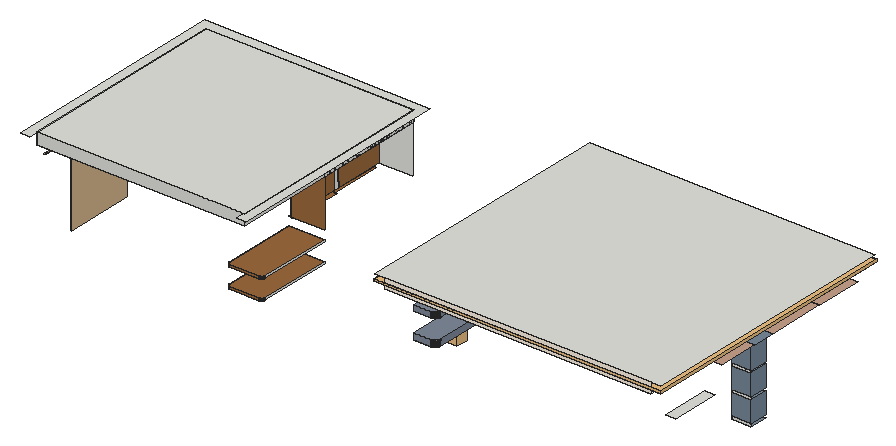
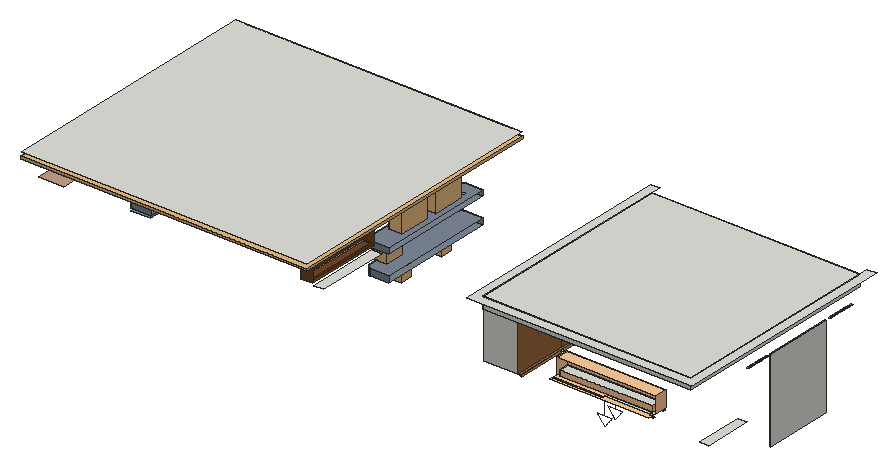
# SketchUp Ruby script. Lengths in inches.
U = 1.inch
M = Sketchup.active_model
def pt(a) = Geom::Point3d.new(a.map { |v| v * U })
def face(e, loops, mat)
  f = e.add_face(loops[0].map { |a| pt(a) })
  loops[1..].each { |l| e.add_face(l.map { |a| pt(a) }).erase! }
  f.material = f.back_material = mat if mat
  f
end
# faces: each face lists its corners as indices into pts; further lists are holes
def faces(e, pts, list, mat = nil) = list.each { |f| face(e, (f[0].is_a?(Array) ? f : [f]).map { |l| l.map { |i| pts[i] } }, mat) }
# xy, xz, yz: faces in a plane at the given z, y or x. An outline is a flat list of corners, or four numbers for a rectangle; further outlines are holes
def ring(l) = l.size == 4 ? [[l[0], l[1]], [l[2], l[1]], [l[2], l[3]], [l[0], l[3]]] : l.each_slice(2).to_a
def flat(e, list, mat, &to3) = list.each { |f| face(e, (f[0].is_a?(Array) ? f : [f]).map { |l| ring(l).map { |u, v| to3.(u, v) } }, mat) }
def xy(e, z, list, mat = nil) = flat(e, list, mat) { |x, y| [x, y, z] }
def xz(e, y, list, mat = nil) = flat(e, list, mat) { |x, z| [x, y, z] }
def yz(e, x, list, mat = nil) = flat(e, list, mat) { |y, z| [x, y, z] }
def lines(e, pts, list) = list.each { |a, b| e.add_line(pt(pts[a]), pt(pts[b])) }
# prism: a flat outline (further loops are holes) pulled along v
def prism(e, loops, v, mat = nil)
  f = face(e, loops, mat); d = Geom::Vector3d.new(v.map { |x| x * U })
  f.pushpull(f.normal.samedirection?(d) ? d.length : -d.length)
end
def box(e, o, s, mat = nil) = prism(e, [[o, [o[0] + s[0], o[1], o[2]], [o[0] + s[0], o[1] + s[1], o[2]], [o[0], o[1] + s[1], o[2]]]], [0, 0, s[2]], mat)
def at(x, y, z, deg = 0) = Geom::Transformation.translation(pt([x, y, z])) * Geom::Transformation.rotation(ORIGIN, Z_AXIS, deg.degrees)
def axes(o, x, y, z) = Geom::Transformation.new([*x, 0, *y, 0, *z, 0, *pt(o).to_a, 1])
def part(name) = M.definitions.add(name)
# library, detail: a bought-in or finely detailed component or shape, given as its bounding box
def library(name, o, s) = part(name).tap { |d| box(d.entities, o, s) }
def detail(e, o, s) = box(e.add_group.entities, o, s)
def put(e, d, t, mat = nil) = e.add_instance(d, t).tap { |i| i.material = mat if mat }
def group(e, t, mat = nil) = e.add_group.tap { |g| g.transformation = t; g.material = mat if mat }.entities
root = M.entities
M.materials.add("Plywood B 50cm").color = [193, 159, 125]
M.materials.add("[0009_Linen]").color = [197, 160, 138]
M.materials.add("[0035_Tan]").color = [210, 180, 140]
M.materials.add("[0110_LightSlateGray]").color = [127, 136, 153]
M.materials.add("[0110_LightSlateGray]1").color = [119, 136, 153]
M.materials.add("[Color C02]").color = [255, 204, 153]
M.materials.add("[Color D01]").color = [255, 242, 228]
M.materials.add("[Fencing Lattice Natural]").color = [179, 148, 127]
M.materials.add("[Wood Floor]").color = [155, 105, 61]
M.materials.add("[Wood Veneer 01]").color = [120, 70, 37]
c1 = library("Spot Light\#1",[-5.1,-5.1,-11.05],[10.2,10.2,11.05])
c2 = library("Spot Light\#3",[-5.1,-5.1,-11.05],[10.2,10.2,11.05])
c3 = library("Spot Light\#2",[-5.1,-5.1,-11.05],[10.2,10.2,11.05])
c4 = part("Group30\#1")
p = [[0,0,0],[0,0,-13.91],[-6.7,0,-13.91],[43.59,-1.45,0],[-43.59,-1.45,0],[43.59,1.45,0],
  [43.59,0,0],[-43.59,1.45,0],[6.7,0,-13.91],[-43.59,0,0],[0,0,-22.52]]
lines(c4.entities,p,[[0,1],[1,2],[3,4],[5,6],[7,5],[1,8],[9,0],[0,6],[8,10],[4,9],[6,3],[2,10],
  [9,7]])
c5 = part("Rectangle Light\#1")
put(c5.entities,c4,at(0,0,0))
c6 = part("Group7\#1")
p = [[0,0,0],[0,0,-13.88],[-6.7,0,-13.88],[43.59,-1.36,0],[-43.59,-1.36,0],[43.59,1.36,0],
  [43.59,0,0],[-43.59,1.36,0],[6.7,0,-13.88],[-43.59,0,0],[0,0,-22.48]]
lines(c6.entities,p,[[0,1],[1,2],[3,4],[5,6],[7,5],[1,8],[9,0],[0,6],[8,10],[4,9],[6,3],[2,10],
  [9,7]])
c7 = part("Rectangle Light")
put(c7.entities,c6,at(0,0,0))
c8 = library("Decorative Puppy 209 004",[-5.43,-3.24,0],[10.86,6.48,10.94])
c9 = library("Books 120 040",[-9.2,-4.08,-0.03],[18.37,8.13,11.52])
c10 = library("Dome Light",[-12,-12,0],[24,24,12])
c11 = library("Mesh Light\#4",[-0.5,-0.5,-0.1],[1,1,0.2])
c12 = library("Group\#10",[-0.5,-0.5,2.25],[131.75,125.15,1.375])
box(root,[8.12,10.37,154.875],[183.2,186.7,9.875])
xy(root,71.0625,[[8.12,47.65,9.43,108.01]])
xy(root,76.9375,[[536.14,116.57,553.2,132.48]],"[0110_LightSlateGray]1")
xy(root,78.9375,[[536.14,116.57,553.2,132.48]],"[0110_LightSlateGray]1")
xy(root,86.125,[[162.88,30.24,162.49,30.26,162.11,30.34,161.73,30.46,161.38,30.64,161.06,30.86,160.76,31.11,160.5,31.41,160.28,31.74,160.11,32.09,159.98,32.46,159.91,32.84,159.88,33.24,159.88,98.61,191.32,98.61,191.32,33.18,191.29,32.79,191.22,32.42,191.1,32.05,190.93,31.71,190.71,31.39,190.46,31.1,190.17,30.84,189.85,30.63,189.5,30.46,189.14,30.34,188.76,30.26,188.38,30.24]],"[Wood Floor]")
xy(root,88.125,[[162.88,30.24,188.38,30.24,188.76,30.26,189.14,30.34,189.5,30.46,189.85,30.63,190.17,30.84,190.46,31.1,190.71,31.39,190.93,31.71,191.1,32.05,191.22,32.42,191.29,32.79,191.32,33.18,191.32,98.61,159.88,98.61,159.88,33.24,159.91,32.84,159.98,32.46,160.11,32.09,160.28,31.74,160.5,31.41,160.76,31.11,161.06,30.86,161.38,30.64,161.73,30.46,162.11,30.34,162.49,30.26]],"[Wood Floor]")
xy(root,98.06,[[536.14,116.57,553.2,132.48]],"[0110_LightSlateGray]1")
xy(root,100.06,[[536.14,116.57,553.2,132.48]],"[0110_LightSlateGray]1")
xy(root,102.15,[[[323.37,31.6,323.37,136.04,338.74,136.04,339.39,136,340.03,135.87,340.65,135.66,341.24,135.37,341.78,135.01,342.28,134.58,342.71,134.09,343.07,133.54,343.36,132.95,343.57,132.34,343.7,131.69,343.74,131.04,343.74,36.6,343.7,35.95,343.57,35.31,343.36,34.69,343.07,34.1,342.71,33.56,342.28,33.07,341.78,32.64,341.24,32.27,340.65,31.98,340.03,31.77,339.39,31.65,338.74,31.6],[335.21,103.85,336.25,103.98,337.21,104.38,338.04,105.02,338.68,105.85,339.07,106.81,339.21,107.85,339.07,108.88,338.68,109.85,338.04,110.67,337.21,111.31,336.25,111.71,335.21,111.85,334.18,111.71,333.21,111.31,332.38,110.67,331.75,109.85,331.35,108.88,331.21,107.85,331.35,106.81,331.75,105.85,332.38,105.02,333.21,104.38,334.18,103.98],[335.41,60.3125,336.29,60.48,337.1,60.87,337.78,61.46,338.28,62.2,338.58,63.05,338.64,63.94,338.48,64.82,338.09,65.63,337.5,66.3125,336.76,66.82,335.91,67.11,335.02,67.18,334.13,67.01,333.33,66.62,332.65,66.03,332.14,65.29,331.85,64.44,331.78,63.55,331.95,62.67,332.34,61.86,332.92,61.18,333.66,60.68,334.51,60.38]]],"[0110_LightSlateGray]")
xy(root,103.09,[[335.21,103.85,334.18,103.98,333.21,104.38,332.38,105.02,331.75,105.85,331.35,106.81,331.21,107.85,331.35,108.88,331.75,109.85,332.38,110.67,333.21,111.31,334.18,111.71,335.21,111.85,336.25,111.71,337.21,111.31,338.04,110.67,338.68,109.85,339.07,108.88,339.21,107.85,339.07,106.81,338.68,105.85,338.04,105.02,337.21,104.38,336.25,103.98]],"[0110_LightSlateGray]")
xy(root,103.5,[[162.88,30.24,162.49,30.26,162.11,30.34,161.73,30.46,161.38,30.64,161.06,30.86,160.76,31.11,160.5,31.41,160.28,31.74,160.11,32.09,159.98,32.46,159.91,32.84,159.88,33.24,159.88,98.61,191.32,98.61,191.32,33.24,191.29,32.84,191.22,32.46,191.09,32.09,190.92,31.74,190.7,31.41,190.44,31.11,190.15,30.86,189.82,30.64,189.47,30.46,189.1,30.34,188.71,30.26,188.32,30.24]],"[Wood Floor]")
xy(root,103.53,[[335.41,60.3125,334.51,60.38,333.66,60.68,332.92,61.18,332.34,61.86,331.95,62.67,331.78,63.55,331.85,64.44,332.14,65.29,332.65,66.03,333.33,66.62,334.13,67.01,335.02,67.18,335.91,67.11,336.76,66.82,337.5,66.3125,338.09,65.63,338.48,64.82,338.64,63.94,338.58,63.05,338.28,62.2,337.78,61.46,337.1,60.87,336.29,60.48]],"[0110_LightSlateGray]")
xy(root,105.5,[[162.88,30.24,188.32,30.24,188.71,30.26,189.1,30.34,189.47,30.46,189.82,30.64,190.15,30.86,190.44,31.11,190.7,31.41,190.92,31.74,191.09,32.09,191.22,32.46,191.29,32.84,191.32,33.24,191.32,98.61,159.88,98.61,159.88,33.24,159.91,32.84,159.98,32.46,160.11,32.09,160.28,31.74,160.5,31.41,160.76,31.11,161.06,30.86,161.38,30.64,161.73,30.46,162.11,30.34,162.49,30.26]],"[Wood Floor]")
xy(root,107.71,[[323.37,31.6,338.74,31.6,339.39,31.65,340.03,31.77,340.65,31.98,341.24,32.27,341.78,32.64,342.28,33.07,342.71,33.56,343.07,34.1,343.36,34.69,343.57,35.31,343.7,35.95,343.74,36.6,343.74,131.04,343.7,131.69,343.57,132.34,343.36,132.95,343.07,133.54,342.71,134.09,342.28,134.58,341.78,135.01,341.24,135.37,340.65,135.66,340.03,135.87,339.39,136,338.74,136.04,323.37,136.04]],"[0110_LightSlateGray]")
xy(root,109.5625,[[0,144.7,8.12,186.76]])
xy(root,110.51,[[159.88,146.875,163.32,147.01]])
xy(root,110.51,[[159.88,101.5625,163.32,109.82],[159.88,109.82,162.26,124.45],[159.88,124.45,163.32,146.875],[159.88,147.01,161.57,192.875]],"[Wood Floor]")
xy(root,113.1875,[[159.88,98.61,161.57,98.61,161.57,146.63,162.01,151.1,162.01,151.32,161.57,146.875,161.57,195.82,159.88,195.82]],"[Wood Floor]")
xy(root,119.18,[[536.14,116.57,553.2,132.48]],"[0110_LightSlateGray]1")
xy(root,121.18,[[536.14,116.57,553.2,132.48]],"[0110_LightSlateGray]1")
xy(root,124.78,[[323.37,31.6,323.37,136.04,338.74,136.04,339.39,136,340.03,135.87,340.65,135.66,341.24,135.37,341.78,135.01,342.28,134.58,342.71,134.09,343.07,133.54,343.36,132.95,343.57,132.34,343.7,131.69,343.74,131.04,343.74,36.6,343.62,35.98,343.43,35.38,343.18,34.8,342.87,34.25,342.5,33.73,342.08,33.26,341.61,32.84,341.1,32.47,340.55,32.16,339.97,31.91,339.36,31.72,338.74,31.6]],"[0110_LightSlateGray]")
xy(root,125.75,[[38.58,199,41.29,200.94]])
xy(root,125.75,[[38.58,186.2,38.58,199,41.29,199,41.29,188.91,123.0625,188.91,123.0625,197.07,41.29,197.07,41.29,200.94,38.58,200.94,38.58,205.19,125.77,205.19,125.77,203.13,80.73,203.13,80.73,200.94,125.77,200.94,125.77,186.2]],"[Color C02]")
xy(root,126.5625,[[41.29,199,80.73,200.94]])
xy(root,129.78,[[[323.37,31.6,338.74,31.6,339.36,31.72,339.97,31.91,340.55,32.16,341.1,32.47,341.61,32.84,342.08,33.26,342.5,33.73,342.87,34.25,343.18,34.8,343.43,35.38,343.62,35.98,343.74,36.6,343.74,131.04,343.7,131.69,343.57,132.34,343.36,132.95,343.07,133.54,342.71,134.09,342.28,134.58,341.78,135.01,341.24,135.37,340.65,135.66,340.03,135.87,339.39,136,338.74,136.04,323.37,136.04],[331.76,41.79,331.08,41.875,330.44,42.14,329.89,42.55,329.47,43.09,329.21,43.72,329.12,44.4,329.2,45.08,329.46,45.72,329.875,46.26,330.41,46.68,331.05,46.95,331.72,47.04,332.4,46.96,333.04,46.7,333.59,46.28,334.01,45.74,334.27,45.11,334.37,44.43,334.28,43.75,334.02,43.12,333.61,42.57,333.07,42.15,332.43,41.88]]],"[0110_LightSlateGray]")
xy(root,130.8125,[[41.29,188.91,123.0625,197.07]])
xy(root,131.66,[[558.07,16.33,566.72,59.9]])
xy(root,136.125,[[314.72,153.92,323.37,217.92]])
xy(root,138.75,[[[323.37,152.04,333.55,219.6],[325.14,153.8125,331.78,217.83]]],"[Wood Veneer 01]")
xy(root,139.75,[[38.58,186.2,125.77,197.07]],"[Color C02]")
xy(root,140.625,[[325.14,153.8125,331.78,217.83]],"[Wood Veneer 01]")
xy(root,142.3,[[536.14,116.57,553.2,132.48]],"[0110_LightSlateGray]1")
xy(root,142.3,[[534.57,116.57,536.14,132.48]],"[Fencing Lattice Natural]")
xy(root,144.0625,[[8.12,18.51,9.37,19.28],[8.12,21,9.37,21.77],[8.12,22.24,9.37,23.01],[8.12,23.49,9.37,24.25],[8.12,24.73,9.37,25.5],
  [8.12,25.98,9.37,26.74],[8.12,27.22,9.37,27.99],[8.12,28.47,9.37,29.23],[8.12,29.71,9.37,30.48],[8.12,30.95,9.37,31.72],
  [8.12,32.2,9.37,32.97],[8.12,33.44,9.37,34.21],[8.12,34.6875,9.37,35.45],[8.12,35.93,9.37,36.7],[8.12,37.18,9.37,37.94],
  [8.12,38.42,9.37,39.1875],[8.12,39.66,9.37,40.43],[8.12,40.91,9.37,41.68],[8.12,42.15,9.37,42.92],[8.12,111.47,9.37,112.23],
  [8.12,112.69,9.37,113.46],[8.12,113.92,9.37,114.6875],[8.12,115.15,9.37,115.91],[8.12,116.375,9.37,117.14],[8.12,117.6,9.37,118.37],
  [8.12,118.83,9.37,119.6],[8.12,120.06,9.37,120.82],[8.12,121.28,9.37,122.05],[8.12,122.51,9.37,123.28],[8.12,123.74,9.37,124.5],
  [8.12,124.97,9.37,125.73],[8.12,126.19,9.37,126.96],[8.12,127.42,9.37,128.1875],[8.12,128.65,9.37,129.41],[8.12,129.875,9.37,130.64],
  [8.12,131.1,9.37,131.87],[8.12,132.33,9.37,133.1]],"Plywood B 50cm")
xy(root,144.0625,[[8.12,47.65,9.43,108.01]],"[0035_Tan]")
xy(root,144.125,[[536.14,78.14,558.07,114.14],[536.14,134.91,558.07,185.66],[536.14,186.26,558.07,228.1]],"[0009_Linen]")
xy(root,144.125,[[536.14,114.74,558.07,134.3125]],"[0110_LightSlateGray]1")
xy(root,152.6875,[[323.37,152.04,333.55,219.6]],"[Wood Veneer 01]")
xy(root,155.0625,[[161.57,98.61,191.32,98.61,191.32,195.82,161.57,195.82,161.57,146.875,162.01,146.875,162.01,146.63,161.57,146.63]],"[Wood Floor]")
xy(root,155.75,[[[323.37,0,558.07,228.1],[378.34,51.98,503.09,51.98,503.49,52,503.87,52.08,504.24,52.21,504.59,52.38,504.92,52.6,505.21,52.86,505.47,53.15,505.69,53.48,505.87,53.83,505.99,54.2,506.07,54.59,506.09,54.98,506.09,176.125,378.34,176.125,377.95,176.1,377.57,176.02,377.2,175.9,376.84,175.72,376.52,175.5,376.22,175.25,375.96,174.95,375.75,174.625,375.57,174.27,375.45,173.9,375.37,173.52,375.34,173.125,375.34,54.98,375.44,54.62,375.57,54.27,375.73,53.93,375.93,53.61,376.15,53.3125,376.4,53.04,376.68,52.79,376.98,52.5625,377.3,52.37,377.63,52.21,377.98,52.08]],[506.09,173.125,506.07,173.52,505.99,173.9,505.87,174.27,505.69,174.625,505.47,174.95,505.21,175.25,504.92,175.5,504.59,175.72,504.24,175.9,503.87,176.02,503.49,176.1,503.09,176.125,506.09,176.125]],"[Color D01]")
xy(root,164.75,[[0,2.25,8.12,2.25,8.12,197.07,191.32,197.07,191.32,98.61,191.13,98.61,191.13,2.25,198.9375,2.25,198.9375,205.19,0,205.19]])
xz(root,0,[[323.37,155.75,558.07,164.75]],"[Color D01]")
xz(root,30.24,[[162.88,86.125,188.38,88.125],[162.88,103.5,188.32,105.5]],"[Wood Floor]")
xz(root,31.6,[[323.37,102.15,338.74,107.71],[323.37,124.78,338.74,129.78]],"[0110_LightSlateGray]")
xz(root,47.65,[[8.12,71.0625,9.43,144.0625]],"[0035_Tan]")
xz(root,51.98,[[378.34,155.75,503.09,158]],"[Color D01]")
xz(root,98.61,[[159.88,86.125,191.32,88.125],[159.88,103.5,191.32,105.5],[191.13,155.0625,191.32,164.75]])
xz(root,98.61,[[161.57,113.1875,191.13,155.0625]],"[Wood Floor]")
xz(root,108.01,[[8.12,71.0625,9.43,144.0625]],"[0035_Tan]")
xz(root,116.57,[[536.14,76.9375,553.2,78.9375],[536.14,98.06,553.2,100.06],[536.14,119.18,553.2,121.18]])
xz(root,116.57,[[536.14,78.9375,553.2,98.06],[536.14,100.06,553.2,119.18],[536.14,121.18,553.2,142.3]],"[0110_LightSlateGray]1")
xz(root,132.48,[[536.14,78.9375,553.2,98.06],[536.14,100.06,553.2,119.18],[536.14,121.18,553.2,142.3]],"[0110_LightSlateGray]1")
xz(root,136.04,[[323.37,102.15,338.74,107.71],[323.37,124.78,338.74,129.78]],"[0110_LightSlateGray]")
xz(root,146.63,[[161.57,113.1875,161.57,155.0625,162.01,155.0625]])
xz(root,146.875,[[161.57,113.1875,162.01,155.0625,161.57,155.0625]])
xz(root,152.04,[[323.37,138.75,333.55,152.6875]],"[Wood Veneer 01]")
xz(root,153.8125,[[325.14,138.75,331.78,140.625]])
xz(root,176.125,[[378.34,155.75,503.09,158]],"[Color D01]")
xz(root,186.2,[[38.58,125.75,125.77,139.75]],"[Color C02]")
xz(root,188.91,[[41.29,125.75,123.0625,130.8125]])
xz(root,195.82,[[161.57,113.1875,191.32,155.0625]])
xz(root,197.07,[[41.29,125.75,123.0625,130.8125]],"[Color C02]")
xz(root,217.83,[[325.14,138.75,331.78,140.625]],"[Wood Veneer 01]")
xz(root,219.6,[[323.37,138.75,333.55,152.6875]],"[Wood Veneer 01]")
yz(root,8.12,[[47.65,71.0625,108.01,144.0625]])
yz(root,9.43,[[47.65,71.0625,108.01,144.0625]],"[0035_Tan]")
yz(root,38.58,[[186.2,125.75,197.07,139.75]],"[Color C02]")
yz(root,41.29,[[199,125.75,200.94,126.5625]])
yz(root,41.29,[[188.91,125.75,197.07,130.8125]],"[Color C02]")
yz(root,123.0625,[[188.91,125.75,197.07,130.8125]])
yz(root,125.77,[[186.2,125.75,197.07,139.75]],"[Color C02]")
yz(root,159.88,[[33.24,86.125,98.61,88.125],[33.24,103.5,98.61,105.5]],"[Wood Floor]")
yz(root,161.57,[[98.61,113.1875,146.63,155.0625],[146.875,113.1875,195.82,155.0625]],"[Wood Floor]")
yz(root,162.01,[[151.1,113.1875,146.63,155.0625,146.875,155.0625,151.32,113.1875]])
yz(root,191.32,[[33.18,86.125,98.61,88.125],[33.24,103.5,98.61,105.5],[98.61,155.0625,195.27,164.75],[195.27,155.0625,195.82,164.75]])
yz(root,325.14,[[153.8125,138.75,217.83,140.625]],"[Wood Veneer 01]")
yz(root,331.78,[[153.8125,138.75,217.83,140.625]])
yz(root,333.55,[[152.04,138.75,219.6,152.6875]],"[Wood Veneer 01]")
yz(root,343.74,[[36.6,102.15,131.04,107.71],[36.6,124.78,131.04,129.78]],"[0110_LightSlateGray]")
yz(root,375.34,[[54.98,155.75,173.125,158]],"[Color D01]")
yz(root,506.09,[[54.98,155.75,173.125,158]],"[Color D01]")
yz(root,536.14,[[116.57,76.9375,132.48,78.9375],[116.57,98.06,132.48,100.06],[116.57,119.18,132.48,121.18]],"[0110_LightSlateGray]1")
yz(root,553.2,[[116.57,78.9375,132.48,98.06],[116.57,100.06,132.48,119.18],[116.57,121.18,132.48,142.3]],"[0110_LightSlateGray]1")
p = [[162.88,30.24,88.125],[162.49,30.26,88.125],[162.49,30.26,86.125],[162.88,30.24,86.125],[188.76,30.26,88.125],[188.38,30.24,88.125],
  [188.38,30.24,86.125],[188.76,30.26,86.125],[162.11,30.34,88.125],[161.73,30.46,88.125],[161.73,30.46,86.125],[162.11,30.34,86.125],
  [189.14,30.34,88.125],[189.14,30.34,86.125],[189.5,30.46,88.125],[189.5,30.46,86.125],[161.38,30.64,88.125],[161.38,30.64,86.125],
  [189.85,30.63,88.125],[189.85,30.63,86.125],[161.06,30.86,88.125],[161.06,30.86,86.125],[190.17,30.84,88.125],[190.17,30.84,86.125],
  [190.46,31.1,88.125],[190.46,31.1,86.125],[160.76,31.11,88.125],[160.76,31.11,86.125],[160.5,31.41,88.125],[160.5,31.41,86.125],
  [190.71,31.39,88.125],[190.71,31.39,86.125],[160.28,31.74,88.125],[160.28,31.74,86.125],[190.93,31.71,88.125],[190.93,31.71,86.125],
  [160.11,32.09,88.125],[160.11,32.09,86.125],[191.1,32.05,88.125],[191.1,32.05,86.125],[159.98,32.46,88.125],[159.98,32.46,86.125],
  [191.22,32.42,88.125],[191.22,32.42,86.125],[191.29,32.79,88.125],[191.29,32.79,86.125],[159.91,32.84,88.125],[159.91,32.84,86.125],
  [159.88,33.24,88.125],[159.88,33.24,86.125],[191.32,33.18,88.125],[191.32,33.18,86.125],[339.39,31.65,107.71],[338.74,31.6,107.71],
  [338.74,31.6,102.15],[339.39,31.65,102.15],[340.03,31.77,107.71],[340.03,31.77,102.15],[340.65,31.98,107.71],[340.65,31.98,102.15],
  [341.24,32.27,107.71],[341.24,32.27,102.15],[341.78,32.64,107.71],[341.78,32.64,102.15],[342.28,33.07,107.71],[342.28,33.07,102.15],
  [342.71,33.56,107.71],[342.71,33.56,102.15],[343.07,34.1,107.71],[343.07,34.1,102.15],[343.36,34.69,107.71],[343.36,34.69,102.15],
  [343.57,35.31,107.71],[343.57,35.31,102.15],[343.7,35.95,107.71],[343.7,35.95,102.15],[343.74,36.6,107.71],[343.74,36.6,102.15],
  [335.41,60.3125,102.15],[334.51,60.38,102.15],[334.51,60.38,103.53],[335.41,60.3125,103.53],[336.29,60.48,102.15],[336.29,60.48,103.53],
  [333.66,60.68,102.15],[333.66,60.68,103.53],[337.1,60.87,102.15],[337.1,60.87,103.53],[332.92,61.18,102.15],[332.92,61.18,103.53],
  [337.78,61.46,102.15],[337.78,61.46,103.53],[332.34,61.86,102.15],[332.34,61.86,103.53],[338.28,62.2,102.15],[338.28,62.2,103.53],
  [331.95,62.67,102.15],[331.95,62.67,103.53],[338.58,63.05,102.15],[338.58,63.05,103.53],[331.78,63.55,102.15],[331.78,63.55,103.53],
  [338.64,63.94,102.15],[338.64,63.94,103.53],[331.85,64.44,102.15],[331.85,64.44,103.53],[338.48,64.82,102.15],[338.48,64.82,103.53],
  [332.14,65.29,102.15],[332.14,65.29,103.53],[338.09,65.63,102.15],[338.09,65.63,103.53],[332.65,66.03,102.15],[332.65,66.03,103.53],
  [337.5,66.3125,102.15],[337.5,66.3125,103.53],[333.33,66.62,102.15],[333.33,66.62,103.53],[336.76,66.82,102.15],[336.76,66.82,103.53],
  [334.13,67.01,102.15],[334.13,67.01,103.53],[335.91,67.11,102.15],[335.91,67.11,103.53],[335.02,67.18,102.15],[335.02,67.18,103.53],
  [335.21,103.85,102.15],[334.18,103.98,102.15],[334.18,103.98,103.09],[335.21,103.85,103.09],[336.25,103.98,102.15],[336.25,103.98,103.09],
  [333.21,104.38,102.15],[333.21,104.38,103.09],[337.21,104.38,102.15],[337.21,104.38,103.09],[332.38,105.02,102.15],[332.38,105.02,103.09],
  [338.04,105.02,102.15],[338.04,105.02,103.09],[331.75,105.85,102.15],[331.75,105.85,103.09],[338.68,105.85,102.15],[338.68,105.85,103.09],
  [331.35,106.81,102.15],[331.35,106.81,103.09],[339.07,106.81,102.15],[339.07,106.81,103.09],[331.21,107.85,102.15],[331.21,107.85,103.09],
  [339.21,107.85,102.15],[339.21,107.85,103.09],[331.35,108.88,102.15],[331.35,108.88,103.09],[339.07,108.88,102.15],[339.07,108.88,103.09],
  [331.75,109.85,102.15],[331.75,109.85,103.09],[338.68,109.85,102.15],[338.68,109.85,103.09],[332.38,110.67,102.15],[332.38,110.67,103.09],
  [338.04,110.67,102.15],[338.04,110.67,103.09],[333.21,111.31,102.15],[333.21,111.31,103.09],[337.21,111.31,102.15],[337.21,111.31,103.09],
  [334.18,111.71,102.15],[334.18,111.71,103.09],[336.25,111.71,102.15],[336.25,111.71,103.09],[335.21,111.85,102.15],[335.21,111.85,103.09],
  [343.7,131.69,107.71],[343.74,131.04,107.71],[343.74,131.04,102.15],[343.7,131.69,102.15],[343.57,132.34,107.71],[343.57,132.34,102.15],
  [343.36,132.95,107.71],[343.36,132.95,102.15],[343.07,133.54,107.71],[343.07,133.54,102.15],[342.71,134.09,107.71],[342.71,134.09,102.15],
  [342.28,134.58,107.71],[342.28,134.58,102.15],[341.78,135.01,107.71],[341.78,135.01,102.15],[341.24,135.37,107.71],[341.24,135.37,102.15],
  [340.65,135.66,107.71],[340.65,135.66,102.15],[340.03,135.87,107.71],[340.03,135.87,102.15],[339.39,136,107.71],[339.39,136,102.15],
  [338.74,136.04,107.71],[338.74,136.04,102.15],[162.88,30.24,105.5],[162.49,30.26,105.5],[162.49,30.26,103.5],[162.88,30.24,103.5],
  [188.71,30.26,105.5],[188.32,30.24,105.5],[188.32,30.24,103.5],[188.71,30.26,103.5],[162.11,30.34,105.5],[161.73,30.46,105.5],
  [161.73,30.46,103.5],[162.11,30.34,103.5],[189.1,30.34,105.5],[189.1,30.34,103.5],[189.47,30.46,105.5],[189.47,30.46,103.5],
  [161.38,30.64,105.5],[161.38,30.64,103.5],[189.82,30.64,105.5],[189.82,30.64,103.5],[161.06,30.86,105.5],[161.06,30.86,103.5],
  [190.15,30.86,105.5],[190.15,30.86,103.5],[160.76,31.11,105.5],[160.76,31.11,103.5],[190.44,31.11,105.5],[190.44,31.11,103.5],
  [160.5,31.41,105.5],[160.5,31.41,103.5],[190.7,31.41,105.5],[190.7,31.41,103.5],[160.28,31.74,105.5],[160.28,31.74,103.5],
  [190.92,31.74,105.5],[190.92,31.74,103.5],[160.11,32.09,105.5],[160.11,32.09,103.5],[191.09,32.09,105.5],[191.09,32.09,103.5],
  [159.98,32.46,105.5],[159.98,32.46,103.5],[191.22,32.46,105.5],[191.22,32.46,103.5],[159.91,32.84,105.5],[159.91,32.84,103.5],
  [191.29,32.84,105.5],[191.29,32.84,103.5],[159.88,33.24,105.5],[159.88,33.24,103.5],[191.32,33.24,105.5],[191.32,33.24,103.5],
  [162.01,151.1,113.1875],[161.57,146.63,113.1875],[162.01,146.63,155.0625],[162.01,151.32,113.1875],[162.01,146.875,155.0625],[161.57,146.875,113.1875],
  [339.36,31.72,129.78],[338.74,31.6,129.78],[338.74,31.6,124.78],[339.36,31.72,124.78],[339.97,31.91,129.78],[339.97,31.91,124.78],
  [340.55,32.16,129.78],[340.55,32.16,124.78],[341.1,32.47,129.78],[341.1,32.47,124.78],[341.61,32.84,129.78],[341.61,32.84,124.78],
  [342.08,33.26,129.78],[342.08,33.26,124.78],[342.5,33.73,129.78],[342.5,33.73,124.78],[342.87,34.25,129.78],[342.87,34.25,124.78],
  [343.18,34.8,129.78],[343.18,34.8,124.78],[343.43,35.38,129.78],[343.43,35.38,124.78],[343.62,35.98,129.78],[343.62,35.98,124.78],
  [343.74,36.6,129.78],[343.74,36.6,124.78],[343.7,131.69,129.78],[343.74,131.04,129.78],[343.74,131.04,124.78],[343.7,131.69,124.78],
  [343.57,132.34,129.78],[343.57,132.34,124.78],[343.36,132.95,129.78],[343.36,132.95,124.78],[343.07,133.54,129.78],[343.07,133.54,124.78],
  [342.71,134.09,129.78],[342.71,134.09,124.78],[342.28,134.58,129.78],[342.28,134.58,124.78],[341.78,135.01,129.78],[341.78,135.01,124.78],
  [341.24,135.37,129.78],[341.24,135.37,124.78],[340.65,135.66,129.78],[340.65,135.66,124.78],[340.03,135.87,129.78],[340.03,135.87,124.78],
  [339.39,136,129.78],[339.39,136,124.78],[338.74,136.04,129.78],[338.74,136.04,124.78],[377.98,52.08,155.75],[377.98,52.08,158],
  [378.34,51.98,158],[378.34,51.98,155.75],[503.09,51.98,155.75],[503.09,51.98,158],[503.49,52,158],[503.49,52,155.75],
  [503.87,52.08,158],[503.87,52.08,155.75],[377.63,52.21,155.75],[377.63,52.21,158],[504.24,52.21,158],[504.24,52.21,155.75],
  [377.3,52.37,155.75],[377.3,52.37,158],[504.59,52.38,158],[504.59,52.38,155.75],[376.98,52.5625,155.75],[376.98,52.5625,158],
  [504.92,52.6,158],[504.92,52.6,155.75],[376.68,52.79,155.75],[376.68,52.79,158],[505.21,52.86,158],[505.21,52.86,155.75],
  [376.4,53.04,155.75],[376.4,53.04,158],[505.47,53.15,158],[505.47,53.15,155.75],[376.15,53.3125,155.75],[376.15,53.3125,158],
  [505.69,53.48,158],[505.69,53.48,155.75],[375.93,53.61,155.75],[375.93,53.61,158],[505.87,53.83,158],[505.87,53.83,155.75],
  [375.73,53.93,155.75],[375.73,53.93,158],[505.99,54.2,158],[505.99,54.2,155.75],[375.57,54.27,155.75],[375.57,54.27,158],
  [506.07,54.59,158],[506.07,54.59,155.75],[375.44,54.62,155.75],[375.44,54.62,158],[375.34,54.98,155.75],[375.34,54.98,158],
  [506.09,54.98,158],[506.09,54.98,155.75],[375.37,173.52,155.75],[375.37,173.52,158],[375.34,173.125,158],[375.34,173.125,155.75],
  [506.09,173.125,155.75],[506.09,173.125,158],[506.07,173.52,158],[506.07,173.52,155.75],[375.45,173.9,155.75],[375.45,173.9,158],
  [505.99,173.9,158],[505.99,173.9,155.75],[375.57,174.27,155.75],[375.57,174.27,158],[505.87,174.27,158],[505.87,174.27,155.75],
  [375.75,174.625,155.75],[375.75,174.625,158],[505.69,174.625,158],[505.69,174.625,155.75],[375.96,174.95,155.75],[375.96,174.95,158],
  [505.47,174.95,158],[505.47,174.95,155.75],[376.22,175.25,155.75],[376.22,175.25,158],[505.21,175.25,158],[505.21,175.25,155.75],
  [376.52,175.5,155.75],[376.52,175.5,158],[504.92,175.5,158],[504.92,175.5,155.75],[376.84,175.72,155.75],[376.84,175.72,158],
  [504.59,175.72,158],[504.59,175.72,155.75],[377.2,175.9,155.75],[377.2,175.9,158],[504.24,175.9,158],[504.24,175.9,155.75],
  [377.57,176.02,155.75],[377.57,176.02,158],[503.87,176.02,158],[503.87,176.02,155.75],[377.95,176.1,155.75],[377.95,176.1,158],
  [503.49,176.1,158],[503.49,176.1,155.75],[378.34,176.125,155.75],[378.34,176.125,158],[503.09,176.125,158],[503.09,176.125,155.75]]
faces(root,p,[[0,1,2,3],[4,5,6,7],[8,9,10,11],[1,8,11,2],[12,4,7,13],[14,12,13,15],[9,16,17,10],[18,14,15,19],
  [16,20,21,17],[22,18,19,23],[24,22,23,25],[20,26,27,21],[26,28,29,27],[30,24,25,31],[28,32,33,29],[34,30,31,35],
  [32,36,37,33],[38,34,35,39],[36,40,41,37],[42,38,39,43],[44,42,43,45],[40,46,47,41],[46,48,49,47],[50,44,45,51],
  [200,201,202,203],[204,205,206,207],[208,209,210,211],[201,208,211,202],[212,204,207,213],[214,212,213,215],[209,216,217,210],[218,214,215,219],
  [216,220,221,217],[222,218,219,223],[220,224,225,221],[226,222,223,227],[224,228,229,225],[230,226,227,231],[228,232,233,229],[234,230,231,235],
  [232,236,237,233],[238,234,235,239],[236,240,241,237],[242,238,239,243],[240,244,245,241],[246,242,243,247],[244,248,249,245],[250,246,247,251]],"[Wood Floor]")
faces(root,p,[[52,53,54,55],[56,52,55,57],[58,56,57,59],[60,58,59,61],[62,60,61,63],[64,62,63,65],[66,64,65,67],[68,66,67,69],
  [70,68,69,71],[72,70,71,73],[74,72,73,75],[76,74,75,77],[78,79,80,81],[82,78,81,83],[79,84,85,80],[86,82,83,87],
  [84,88,89,85],[90,86,87,91],[88,92,93,89],[94,90,91,95],[92,96,97,93],[98,94,95,99],[96,100,101,97],[102,98,99,103],
  [100,104,105,101],[106,102,103,107],[104,108,109,105],[110,106,107,111],[108,112,113,109],[114,110,111,115],[112,116,117,113],[118,114,115,119],
  [116,120,121,117],[122,118,119,123],[120,124,125,121],[124,122,123,125],[126,127,128,129],[130,126,129,131],[127,132,133,128],[134,130,131,135],
  [132,136,137,133],[138,134,135,139],[136,140,141,137],[142,138,139,143],[140,144,145,141],[146,142,143,147],[144,148,149,145],[150,146,147,151],
  [148,152,153,149],[154,150,151,155],[152,156,157,153],[158,154,155,159],[156,160,161,157],[162,158,159,163],[160,164,165,161],[166,162,163,167],
  [164,168,169,165],[170,166,167,171],[168,172,173,169],[172,170,171,173],[174,175,176,177],[178,174,177,179],[180,178,179,181],[182,180,181,183],
  [184,182,183,185],[186,184,185,187],[188,186,187,189],[190,188,189,191],[192,190,191,193],[194,192,193,195],[196,194,195,197],[198,196,197,199],
  [258,259,260,261],[262,258,261,263],[264,262,263,265],[266,264,265,267],[268,266,267,269],[270,268,269,271],[272,270,271,273],[274,272,273,275],
  [276,274,275,277],[278,276,277,279],[280,278,279,281],[282,280,281,283],[284,285,286,287],[288,284,287,289],[290,288,289,291],[292,290,291,293],
  [294,292,293,295],[296,294,295,297],[298,296,297,299],[300,298,299,301],[302,300,301,303],[304,302,303,305],[306,304,305,307],[308,306,307,309]],"[0110_LightSlateGray]")
faces(root,p,[[252,253,254],[255,256,257]])
faces(root,p,[[310,311,312,313],[314,315,316,317],[317,316,318,319],[320,321,311,310],[319,318,322,323],[324,325,321,320],[323,322,326,327],[328,329,325,324],
  [327,326,330,331],[332,333,329,328],[331,330,334,335],[336,337,333,332],[335,334,338,339],[340,341,337,336],[339,338,342,343],[344,345,341,340],
  [343,342,346,347],[348,349,345,344],[347,346,350,351],[352,353,349,348],[351,350,354,355],[356,357,353,352],[358,359,357,356],[355,354,360,361],
  [362,363,364,365],[366,367,368,369],[370,371,363,362],[369,368,372,373],[374,375,371,370],[373,372,376,377],[378,379,375,374],[377,376,380,381],
  [382,383,379,378],[381,380,384,385],[386,387,383,382],[385,384,388,389],[390,391,387,386],[389,388,392,393],[394,395,391,390],[393,392,396,397],
  [398,399,395,394],[397,396,400,401],[402,403,399,398],[401,400,404,405],[406,407,403,402],[405,404,408,409],[410,411,407,406],[409,408,412,413]],"[Color D01]")
detail(root,[380.47,57.11,155.75],[120.49,113.89,3.625])
put(root,c1,at(542.65,124.62,96.68))
put(root,c2,at(334.52,109.18,101.45))
put(root,c3,at(335.21,63.75,101.95))
put(root,c5,at(82.18,187.65,124.05))
put(root,c7,at(80.73,200.94,124.6875))
put(root,c8,axes([340.59,115.5,107.71],[0,1.5444,0],[-1.8876,0,0],[0,0,1.43]))
put(root,c1,at(542.65,124.62,119.18))
put(root,c9,axes([334.55,63.91,129.5],[0,1.5,0],[-1.5,0,0],[0,0,1.5]))
put(root,c9,axes([334.45,100.91,129.73],[0,1.5,0],[-1.5,0,0],[0,0,1.5]))
put(root,c1,at(542.65,124.62,141.35))
put(root,c10,axes([106.71,109.24,132.38],[1.8744,0,0],[0,1.8744,0],[0,0,1.8744]))
put(root,c10,axes([60.09,109.24,132.38],[1.8744,0,0],[0,1.8744,0],[0,0,1.8744]))
g1 = group(root,at(314.72,0,155.75))
xy(g1,3.625,[[[63.625,51.98,63.26,52.08,62.91,52.21,62.58,52.37,62.26,52.5625,61.96,52.79,61.68,53.04,61.43,53.3125,61.21,53.61,61.01,53.93,60.85,54.27,60.72,54.62,60.625,54.98,60.625,173.125,60.65,173.52,60.73,173.9,60.85,174.27,61.03,174.625,61.25,174.95,61.5,175.25,61.8,175.5,62.125,175.72,62.48,175.9,62.85,176.02,63.23,176.1,63.625,176.125,188.375,176.125,188.77,176.1,189.15,176.02,189.52,175.9,189.875,175.72,190.2,175.5,190.5,175.25,190.75,174.95,190.97,174.625,191.15,174.27,191.27,173.9,191.35,173.52,191.375,173.125,191.375,54.98,191.35,54.59,191.27,54.2,191.15,53.83,190.97,53.48,190.75,53.15,190.5,52.86,190.2,52.6,189.875,52.38,189.52,52.21,189.15,52.08,188.77,52,188.375,51.98],[68.75,57.11,183.25,57.11,183.64,57.13,184.02,57.21,184.39,57.34,184.75,57.51,185.07,57.73,185.37,57.99,185.625,58.28,185.84,58.61,186.02,58.96,186.14,59.33,186.22,59.72,186.25,60.11,186.25,171,68.75,171,68.36,170.97,67.98,170.89,67.61,170.77,67.25,170.59,66.93,170.375,66.63,170.12,66.375,169.82,66.16,169.5,65.98,169.14,65.86,168.77,65.78,168.39,65.75,168,65.75,60.11,65.78,59.72,65.86,59.33,65.98,58.96,66.16,58.61,66.375,58.28,66.63,57.99,66.93,57.73,67.25,57.51,67.61,57.34,67.98,57.21,68.36,57.13]]],"[Color D01]")
xy(g1,9,[[0,0,252,236.75]])
yz(g1,65.75,[[60.11,0,168,3.625]],"[Color D01]")
p = [[84.82,148.93,0],[84.82,149.4,0]]
lines(g1,p,[[0,1]])
detail(g1,[84.82,76.17,0],[82.36,75.76,0.8125])
put(g1,c11,axes([126,118.375,4.5],[253,0,0],[0,237.75,0],[0,0,10]))
put(root,c12,at(375.34,51.98,155.75))
